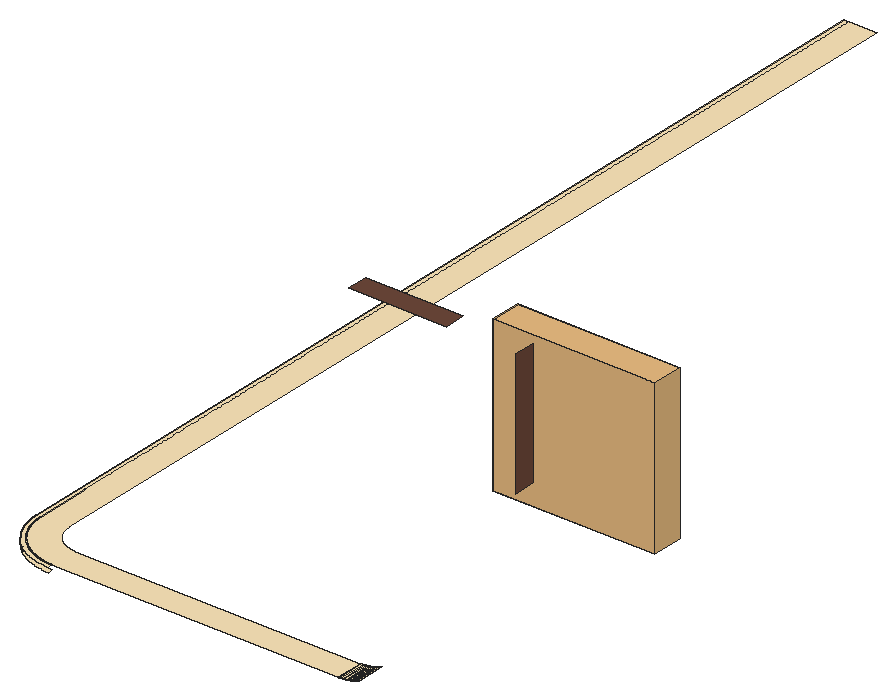
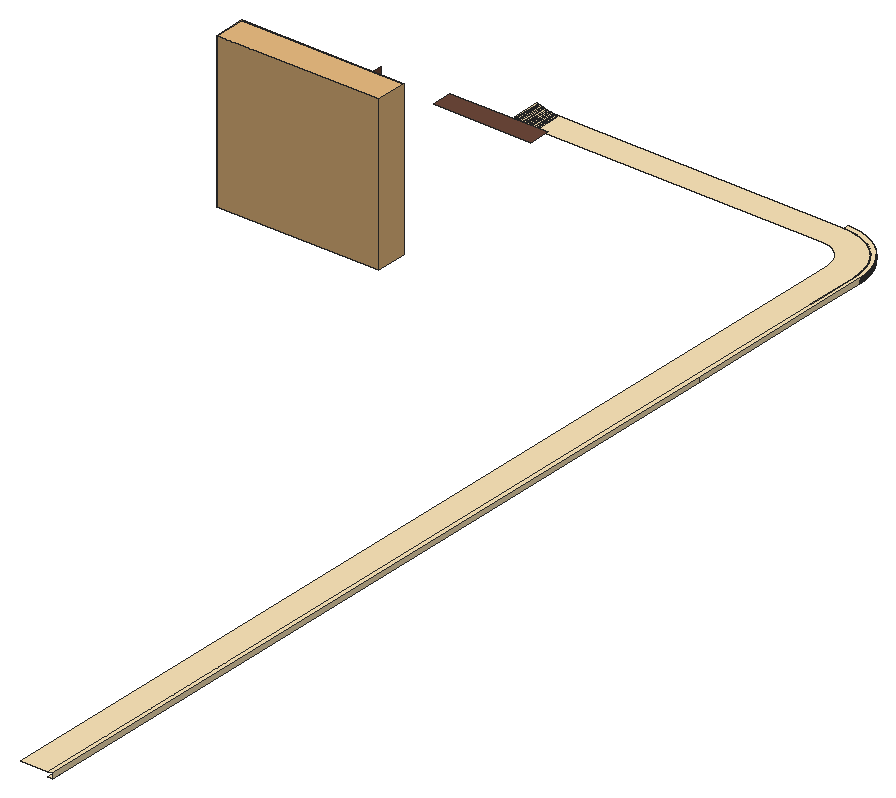
# SketchUp Ruby script. Lengths in inches.
U = 1.inch
M = Sketchup.active_model
def pt(a) = Geom::Point3d.new(a.map { |v| v * U })
def face(e, loops, mat)
  f = e.add_face(loops[0].map { |a| pt(a) })
  loops[1..].each { |l| e.add_face(l.map { |a| pt(a) }).erase! }
  f.material = f.back_material = mat if mat
  f
end
# faces: each face lists its corners as indices into pts; further lists are holes
def faces(e, pts, list, mat = nil) = list.each { |f| face(e, (f[0].is_a?(Array) ? f : [f]).map { |l| l.map { |i| pts[i] } }, mat) }
# xy, xz, yz: faces in a plane at the given z, y or x. An outline is a flat list of corners, or four numbers for a rectangle; further outlines are holes
def ring(l) = l.size == 4 ? [[l[0], l[1]], [l[2], l[1]], [l[2], l[3]], [l[0], l[3]]] : l.each_slice(2).to_a
def flat(e, list, mat, &to3) = list.each { |f| face(e, (f[0].is_a?(Array) ? f : [f]).map { |l| ring(l).map { |u, v| to3.(u, v) } }, mat) }
def xy(e, z, list, mat = nil) = flat(e, list, mat) { |x, y| [x, y, z] }
def xz(e, y, list, mat = nil) = flat(e, list, mat) { |x, z| [x, y, z] }
def yz(e, x, list, mat = nil) = flat(e, list, mat) { |y, z| [x, y, z] }
def lines(e, pts, list) = list.each { |a, b| e.add_line(pt(pts[a]), pt(pts[b])) }
# prism: a flat outline (further loops are holes) pulled along v
def prism(e, loops, v, mat = nil)
  f = face(e, loops, mat); d = Geom::Vector3d.new(v.map { |x| x * U })
  f.pushpull(f.normal.samedirection?(d) ? d.length : -d.length)
end
def box(e, o, s, mat = nil) = prism(e, [[o, [o[0] + s[0], o[1], o[2]], [o[0] + s[0], o[1] + s[1], o[2]], [o[0], o[1] + s[1], o[2]]]], [0, 0, s[2]], mat)
def at(x, y, z, deg = 0) = Geom::Transformation.translation(pt([x, y, z])) * Geom::Transformation.rotation(ORIGIN, Z_AXIS, deg.degrees)
def axes(o, x, y, z) = Geom::Transformation.new([*x, 0, *y, 0, *z, 0, *pt(o).to_a, 1])
def part(name) = M.definitions.add(name)
# library, detail: a bought-in or finely detailed component or shape, given as its bounding box
def library(name, o, s) = part(name).tap { |d| box(d.entities, o, s) }
def detail(e, o, s) = box(e.add_group.entities, o, s)
def put(e, d, t, mat = nil) = e.add_instance(d, t).tap { |i| i.material = mat if mat }
def group(e, t, mat = nil) = e.add_group.tap { |g| g.transformation = t; g.material = mat if mat }.entities
root = M.entities
M.materials.add("1026 AP 7946 SUNNY SIDE UP").color = [254, 231, 186]
M.materials.add("1916 AP K226 Macadamia Cream-N").color = [109, 72, 58]
c1 = library("---------1\#1",[5.49,6.625,-77.21],[69.81,13.39,114.05])
xy(root,142,[[29.49,213.1,28.99,213.12,28.73,213.13,28.48,213.14,27.98,213.18,27.72,213.2,27.47,213.22,26.72,213.31,26.46,213.34,25.46,213.5,25.21,213.55,24.97,213.59,24.72,213.65,24.22,213.75,23.98,213.8125,23.73,213.87,23.48,213.93,23.24,214,22.99,214.07,22.27,214.28,22.02,214.36,21.54,214.52,21.31,214.61,21.07,214.69,20.59,214.87,20.36,214.97,20.125,215.0625,19.89,215.16,19.43,215.36,19.19,215.47,18.96,215.57,18.74,215.68,18.51,215.8,18.28,215.91,18.06,216.02,17.83,216.14,17.61,216.26,17.39,216.39,17.17,216.51,16.51,216.9,16.3,217.03,16.08,217.17,15.87,217.3,15.66,217.44,15.45,217.59,15.24,217.73,15.03,217.875,14.83,218.02,14.42,218.32,14.22,218.48,14.02,218.63,13.82,218.79,13.43,219.11,13.24,219.28,13.04,219.44,12.66,219.78,12.48,219.95,12.29,220.12,12.11,220.3,11.93,220.47,11.39,221.01,11.22,221.2,11.04,221.38,10.53,221.95,10.21,222.33,10.04,222.53,9.88,222.72,9.73,222.92,9.57,223.12,9.42,223.32,9.26,223.52,9.11,223.73,8.96,223.93,8.82,224.14,8.67,224.35,8.25,224.98,8.12,225.2,7.99,225.41,7.85,225.63,7.72,225.84,7.6,226.0625,7.47,226.28,7.35,226.51,7.11,226.95,6.99,227.18,6.88,227.4,6.44,228.32,6.24,228.78,6.14,229.02,6.05,229.25,5.95,229.49,5.86,229.72,5.68,230.2,5.6,230.4375,5.52,230.68,5.4375,230.92,5.36,231.16,5.29,231.4,5.21,231.64,5.14,231.89,5.07,232.13,4.95,232.62,4.88,232.87,4.83,233.11,4.77,233.36,4.67,233.86,4.62,234.1,4.57,234.35,4.41,235.35,4.38,235.61,4.29,236.36,4.27,236.61,4.24,236.87,4.23,237.12,4.21,237.37,4.19,237.625,4.18,237.875,4.17,238.13,4.17,238.38,4.16,238.64,4.12,262.95,6,262.9375,6.16,238.66,6.17,238.43,6.17,238.19,6.19,237.73,6.21,237.49,6.22,237.26,6.24,237.03,6.26,236.79,6.3,236.33,6.33,236.1,6.36,235.86,6.39,235.63,6.43,235.4,6.46,235.17,6.5,234.9375,6.54,234.71,6.58,234.48,6.67,234.02,6.72,233.79,6.77,233.5625,6.83,233.34,6.88,233.11,6.94,232.88,7,232.66,7.07,232.43,7.13,232.21,7.2,231.98,7.41,231.32,7.49,231.09,7.57,230.875,7.65,230.65,7.73,230.4375,7.8125,230.22,7.9,230,7.99,229.78,8.08,229.57,8.17,229.35,8.27,229.14,8.36,228.93,8.56,228.51,8.67,228.3,8.77,228.09,8.99,227.67,9.1,227.47,9.22,227.26,9.33,227.06,9.57,226.66,9.6875,226.46,9.8125,226.26,9.9375,226.0625,10.07,225.87,10.19,225.67,10.33,225.48,10.46,225.28,10.59,225.09,10.73,224.9,10.87,224.72,11.15,224.34,11.29,224.16,11.74,223.62,11.89,223.4375,12.04,223.26,12.2,223.09,12.35,222.91,12.99,222.23,13.16,222.07,13.49,221.74,13.83,221.42,14.01,221.26,14.18,221.1,14.36,220.95,14.53,220.8,15.07,220.35,15.26,220.21,15.44,220.0625,15.625,219.92,16,219.64,16.19,219.51,16.38,219.37,16.58,219.24,16.96,218.98,17.16,218.85,17.36,218.73,17.56,218.6,17.96,218.36,18.16,218.25,18.36,218.13,18.57,218.02,18.77,217.91,18.98,217.8,19.1875,217.69,19.4,217.59,19.61,217.48,20.03,217.28,20.24,217.1875,20.46,217.09,20.67,217,20.89,216.91,21.1,216.82,21.32,216.74,21.54,216.65,22.2,216.41,22.42,216.34,22.64,216.26,22.86,216.19,23.09,216.125,23.3125,216.06,23.54,215.99,23.76,215.93,23.99,215.87,24.21,215.8125,24.44,215.76,24.67,215.7,24.9,215.65,25.125,215.6,25.35,215.56,25.58,215.51,25.8125,215.47,26.04,215.43,26.28,215.39,26.51,215.36,26.74,215.32,27.2,215.26,27.43,215.24,27.67,215.21,28.13,215.17,28.36,215.16,28.6,215.14,28.83,215.13,29.07,215.12,29.53,215.1,29.77,215.1,29.76,215,29.75,213.1],[6,262.9375,4.12,262.95,4,325.89,4,674,6,674]],"1026 AP 7946 SUNNY SIDE UP")
xy(root,144,[[29.49,213.1,29.75,213.1,29.76,215,29.53,215,29.29,215.01,29.06,215.02,28.82,215.03,28.59,215.04,28.35,215.06,28.12,215.07,27.88,215.09,27.65,215.12,27.42,215.14,27.18,215.17,26.95,215.19,26.72,215.23,26.48,215.26,26.25,215.29,25.79,215.37,25.55,215.42,25.32,215.46,24.4,215.66,24.18,215.72,23.49,215.9,23.27,215.96,23.04,216.03,22.82,216.1,22.59,216.17,22.37,216.25,22.15,216.32,21.92,216.4,21.7,216.48,21.48,216.5625,21.26,216.65,21.04,216.73,20.83,216.82,20.61,216.91,20.39,217.01,20.18,217.1,19.96,217.2,19.33,217.5,18.7,217.83,18.49,217.9375,18.29,218.05,18.08,218.17,17.67,218.41,17.27,218.65,17.07,218.78,16.68,219.04,16.48,219.17,16.29,219.3,16.1,219.4375,15.91,219.57,15.53,219.85,15.34,220,15.16,220.14,14.97,220.29,14.25,220.89,14.07,221.05,13.9,221.2,13.72,221.36,13.38,221.68,13.21,221.85,13.04,222.01,12.88,222.18,12.71,222.35,12.39,222.69,12.23,222.87,12.08,223.04,11.92,223.22,11.77,223.39,11.61,223.57,11.46,223.76,11.31,223.9375,11.17,224.12,11.02,224.31,10.88,224.49,10.6,224.87,10.46,225.0625,10.33,225.25,10.19,225.45,10.06,225.64,9.8,226.04,9.68,226.24,9.55,226.44,9.19,227.04,9.07,227.25,8.96,227.45,8.52,228.29,8.22,228.92,8.12,229.14,8.02,229.35,7.93,229.57,7.84,229.78,7.66,230.22,7.58,230.44,7.49,230.66,7.41,230.88,7.34,231.1,7.26,231.33,7.19,231.55,7.11,231.77,7.04,232,6.98,232.22,6.91,232.45,6.85,232.68,6.79,232.9,6.67,233.36,6.42,234.51,6.34,234.97,6.3,235.21,6.27,235.4375,6.23,235.67,6.2,235.9,6.17,236.14,6.14,236.37,6.12,236.61,6.1,236.84,6.08,237.08,6.04,237.54,6.03,237.78,6.02,238.01,6,238.49,6,674,4,674,4,325.89,4.16,238.64,4.17,238.38,4.17,238.13,4.18,237.875,4.19,237.625,4.21,237.37,4.23,237.12,4.24,236.87,4.27,236.61,4.29,236.36,4.38,235.61,4.41,235.35,4.57,234.35,4.62,234.1,4.67,233.86,4.77,233.36,4.83,233.11,4.88,232.87,4.95,232.62,5.07,232.13,5.14,231.89,5.21,231.64,5.29,231.4,5.36,231.16,5.4375,230.92,5.52,230.68,5.6,230.4375,5.68,230.2,5.86,229.72,5.95,229.49,6.05,229.25,6.14,229.02,6.24,228.78,6.44,228.32,6.88,227.4,6.99,227.18,7.11,226.95,7.35,226.51,7.47,226.28,7.6,226.0625,7.72,225.84,7.85,225.63,7.99,225.41,8.12,225.2,8.25,224.98,8.67,224.35,8.82,224.14,8.96,223.93,9.11,223.73,9.26,223.52,9.42,223.32,9.57,223.12,9.73,222.92,9.88,222.72,10.04,222.53,10.21,222.33,10.53,221.95,11.04,221.38,11.22,221.2,11.39,221.01,11.93,220.47,12.11,220.3,12.29,220.12,12.48,219.95,12.66,219.78,13.04,219.44,13.24,219.28,13.43,219.11,13.82,218.79,14.02,218.63,14.22,218.48,14.42,218.32,14.83,218.02,15.03,217.875,15.24,217.73,15.45,217.59,15.66,217.44,15.87,217.3,16.08,217.17,16.3,217.03,16.51,216.9,17.17,216.51,17.39,216.39,17.61,216.26,17.83,216.14,18.06,216.02,18.28,215.91,18.51,215.8,18.74,215.68,18.96,215.57,19.19,215.47,19.43,215.36,19.89,215.16,20.125,215.0625,20.36,214.97,20.59,214.87,21.07,214.69,21.31,214.61,21.54,214.52,22.02,214.36,22.27,214.28,22.99,214.07,23.24,214,23.48,213.93,23.73,213.87,23.98,213.8125,24.22,213.75,24.72,213.65,24.97,213.59,25.21,213.55,25.46,213.5,26.46,213.34,26.72,213.31,27.47,213.22,27.72,213.2,27.98,213.18,28.48,213.14,28.73,213.13,28.99,213.12],[29.53,215,29.76,215,29.77,215.1,29.53,215.1,29.07,215.12,28.83,215.13,28.6,215.14,28.36,215.16,28.13,215.17,27.67,215.21,27.43,215.24,27.2,215.26,26.74,215.32,26.51,215.36,26.28,215.39,26.04,215.43,25.8125,215.47,25.58,215.51,25.35,215.56,25.125,215.6,24.9,215.65,24.67,215.7,24.44,215.76,24.21,215.8125,23.99,215.87,23.76,215.93,23.54,215.99,23.3125,216.06,23.09,216.125,22.86,216.19,22.64,216.26,22.42,216.34,22.2,216.41,21.54,216.65,21.32,216.74,21.1,216.82,20.89,216.91,20.67,217,20.46,217.09,20.24,217.1875,20.03,217.28,19.61,217.48,19.4,217.59,19.1875,217.69,18.98,217.8,18.77,217.91,18.57,218.02,18.36,218.13,18.16,218.25,17.96,218.36,17.56,218.6,17.36,218.73,17.16,218.85,16.96,218.98,16.58,219.24,16.38,219.37,16.19,219.51,16,219.64,15.625,219.92,15.44,220.0625,15.26,220.21,15.07,220.35,14.53,220.8,14.36,220.95,14.18,221.1,14.01,221.26,13.83,221.42,13.49,221.74,13.16,222.07,12.99,222.23,12.35,222.91,12.2,223.09,12.04,223.26,11.89,223.4375,11.74,223.62,11.29,224.16,11.15,224.34,10.87,224.72,10.73,224.9,10.59,225.09,10.46,225.28,10.33,225.48,10.19,225.67,10.07,225.87,9.9375,226.0625,9.8125,226.26,9.6875,226.46,9.57,226.66,9.33,227.06,9.22,227.26,9.1,227.47,8.99,227.67,8.77,228.09,8.67,228.3,8.56,228.51,8.36,228.93,8.27,229.14,8.17,229.35,8.08,229.57,7.99,229.78,7.9,230,7.8125,230.22,7.73,230.4375,7.65,230.65,7.57,230.875,7.49,231.09,7.41,231.32,7.2,231.98,7.13,232.21,7.07,232.43,7,232.66,6.94,232.88,6.88,233.11,6.83,233.34,6.77,233.5625,6.72,233.79,6.67,234.02,6.58,234.48,6.54,234.71,6.5,234.9375,6.46,235.17,6.43,235.4,6.39,235.63,6.36,235.86,6.33,236.1,6.3,236.33,6.26,236.79,6.24,237.03,6.22,237.26,6.21,237.49,6.19,237.73,6.17,238.19,6.17,238.43,6.16,238.66,6,262.9375,6,238.49,6.02,238.01,6.03,237.78,6.04,237.54,6.08,237.08,6.1,236.84,6.12,236.61,6.14,236.37,6.17,236.14,6.2,235.9,6.23,235.67,6.27,235.4375,6.3,235.21,6.34,234.97,6.42,234.51,6.67,233.36,6.79,232.9,6.85,232.68,6.91,232.45,6.98,232.22,7.04,232,7.11,231.77,7.19,231.55,7.26,231.33,7.34,231.1,7.41,230.88,7.49,230.66,7.58,230.44,7.66,230.22,7.84,229.78,7.93,229.57,8.02,229.35,8.12,229.14,8.22,228.92,8.52,228.29,8.96,227.45,9.07,227.25,9.19,227.04,9.55,226.44,9.68,226.24,9.8,226.04,10.06,225.64,10.19,225.45,10.33,225.25,10.46,225.0625,10.6,224.87,10.88,224.49,11.02,224.31,11.17,224.12,11.31,223.9375,11.46,223.76,11.61,223.57,11.77,223.39,11.92,223.22,12.08,223.04,12.23,222.87,12.39,222.69,12.71,222.35,12.88,222.18,13.04,222.01,13.21,221.85,13.38,221.68,13.72,221.36,13.9,221.2,14.07,221.05,14.25,220.89,14.97,220.29,15.16,220.14,15.34,220,15.53,219.85,15.91,219.57,16.1,219.4375,16.29,219.3,16.48,219.17,16.68,219.04,17.07,218.78,17.27,218.65,17.67,218.41,18.08,218.17,18.29,218.05,18.49,217.9375,18.7,217.83,19.33,217.5,19.96,217.2,20.18,217.1,20.39,217.01,20.61,216.91,20.83,216.82,21.04,216.73,21.26,216.65,21.48,216.5625,21.7,216.48,21.92,216.4,22.15,216.32,22.37,216.25,22.59,216.17,22.82,216.1,23.04,216.03,23.27,215.96,23.49,215.9,24.18,215.72,24.4,215.66,25.32,215.46,25.55,215.42,25.79,215.37,26.25,215.29,26.48,215.26,26.72,215.23,26.95,215.19,27.18,215.17,27.42,215.14,27.65,215.12,27.88,215.09,28.12,215.07,28.35,215.06,28.59,215.04,28.82,215.03,29.06,215.02,29.29,215.01],[29.53,215.1,153,215.1,153,227,29.81,227,29.53,227.01,29.29,227.02,29.06,227.04,28.82,227.06,28.59,227.08,28.36,227.11,28.01,227.17,27.77,227.21,27.54,227.25,27.3125,227.3,27.08,227.36,26.86,227.42,26.63,227.48,26.52,227.52,26.18,227.625,25.96,227.7,25.74,227.78,25.08,228.05,24.66,228.25,24.24,228.47,24.03,228.59,23.63,228.83,23.43,228.96,23.24,229.09,23.04,229.22,22.66,229.5,22.48,229.65,22.39,229.72,22.03,230.03,21.85,230.1875,21.68,230.35,21.35,230.68,21.1875,230.85,21.03,231.03,20.72,231.39,20.58,231.57,20.43,231.76,20.36,231.85,20.22,232.04,20.15,232.14,20.02,232.33,19.89,232.53,19.65,232.93,19.53,233.14,19.47,233.24,19.36,233.45,19.2,233.76,19.15,233.87,19.05,234.08,18.78,234.74,18.66,235.07,18.55,235.4,18.52,235.52,18.45,235.74,18.42,235.86,18.36,236.08,18.3,236.3125,18.25,236.54,18.23,236.66,18.1875,236.89,18.17,237.01,18.11,237.36,18.08,237.59,18.06,237.82,18.04,238.06,18.02,238.29,18.01,238.53,18,238.76,18,674,6,674,6,262.9375,6.16,238.66,6.17,238.43,6.17,238.19,6.19,237.73,6.21,237.49,6.22,237.26,6.24,237.03,6.26,236.79,6.3,236.33,6.33,236.1,6.36,235.86,6.39,235.63,6.43,235.4,6.46,235.17,6.5,234.9375,6.54,234.71,6.58,234.48,6.67,234.02,6.72,233.79,6.77,233.5625,6.83,233.34,6.88,233.11,6.94,232.88,7,232.66,7.07,232.43,7.13,232.21,7.2,231.98,7.41,231.32,7.49,231.09,7.57,230.875,7.65,230.65,7.73,230.4375,7.8125,230.22,7.9,230,7.99,229.78,8.08,229.57,8.17,229.35,8.27,229.14,8.36,228.93,8.56,228.51,8.67,228.3,8.77,228.09,8.99,227.67,9.1,227.47,9.22,227.26,9.33,227.06,9.57,226.66,9.6875,226.46,9.8125,226.26,9.9375,226.0625,10.07,225.87,10.19,225.67,10.33,225.48,10.46,225.28,10.59,225.09,10.73,224.9,10.87,224.72,11.15,224.34,11.29,224.16,11.74,223.62,11.89,223.4375,12.04,223.26,12.2,223.09,12.35,222.91,12.99,222.23,13.16,222.07,13.49,221.74,13.83,221.42,14.01,221.26,14.18,221.1,14.36,220.95,14.53,220.8,15.07,220.35,15.26,220.21,15.44,220.0625,15.625,219.92,16,219.64,16.19,219.51,16.38,219.37,16.58,219.24,16.96,218.98,17.16,218.85,17.36,218.73,17.56,218.6,17.96,218.36,18.16,218.25,18.36,218.13,18.57,218.02,18.77,217.91,18.98,217.8,19.1875,217.69,19.4,217.59,19.61,217.48,20.03,217.28,20.24,217.1875,20.46,217.09,20.67,217,20.89,216.91,21.1,216.82,21.32,216.74,21.54,216.65,22.2,216.41,22.42,216.34,22.64,216.26,22.86,216.19,23.09,216.125,23.3125,216.06,23.54,215.99,23.76,215.93,23.99,215.87,24.21,215.8125,24.44,215.76,24.67,215.7,24.9,215.65,25.125,215.6,25.35,215.56,25.58,215.51,25.8125,215.47,26.04,215.43,26.28,215.39,26.51,215.36,26.74,215.32,27.2,215.26,27.43,215.24,27.67,215.21,28.13,215.17,28.36,215.16,28.6,215.14,28.83,215.13,29.07,215.12],[153,215.1,153.24,227],[153.24,215.1,153.47,227]],"1026 AP 7946 SUNNY SIDE UP")
xy(root,216,[[69,326,111,335]],"1916 AP K226 Macadamia Cream-N")
yz(root,4,[[325.89,142,674,144]],"1026 AP 7946 SUNNY SIDE UP")
yz(root,4.17,[[238.13,142,238.38,144]],"1026 AP 7946 SUNNY SIDE UP")
yz(root,6.17,[[238.19,142,238.43,144]],"1026 AP 7946 SUNNY SIDE UP")
yz(root,141,[[326,162,335,216]],"1916 AP K226 Macadamia Cream-N")
p = [[17.96,218.36,142],[17.96,218.36,144],[18.16,218.25,144],[18.16,218.25,142],[14.22,218.48,144],[14.22,218.48,142],
  [14.42,218.32,142],[14.42,218.32,144],[17.76,218.48,142],[17.76,218.48,144],[14.02,218.63,144],[14.02,218.63,142],
  [17.56,218.6,142],[17.56,218.6,144],[13.82,218.79,144],[13.82,218.79,142],[17.36,218.73,142],[17.36,218.73,144],
  [17.16,218.85,142],[17.16,218.85,144],[13.625,218.95,144],[13.625,218.95,142],[16.96,218.98,142],[16.96,218.98,144],
  [13.43,219.11,144],[13.43,219.11,142],[16.77,219.11,142],[16.77,219.11,144],[13.24,219.28,144],[13.24,219.28,142],
  [16.58,219.24,142],[16.58,219.24,144],[16.38,219.37,142],[16.38,219.37,144],[13.04,219.44,144],[13.04,219.44,142],
  [12.85,219.61,144],[12.85,219.61,142],[16.19,219.51,142],[16.19,219.51,144],[16,219.64,142],[16,219.64,144],
  [12.66,219.78,144],[12.66,219.78,142],[15.8125,219.78,142],[15.8125,219.78,144],[12.48,219.95,144],[12.48,219.95,142],
  [15.625,219.92,142],[15.625,219.92,144],[12.29,220.12,144],[12.29,220.12,142],[15.44,220.0625,142],[15.44,220.0625,144],
  [12.11,220.3,144],[12.11,220.3,142],[15.26,220.21,142],[15.26,220.21,144],[15.07,220.35,142],[15.07,220.35,144],
  [11.93,220.47,144],[11.93,220.47,142],[14.89,220.5,142],[14.89,220.5,144],[11.75,220.65,144],[11.75,220.65,142],
  [14.71,220.65,142],[14.71,220.65,144],[14.53,220.8,142],[14.53,220.8,144],[11.57,220.83,144],[11.57,220.83,142],
  [11.39,221.01,144],[11.39,221.01,142],[14.36,220.95,142],[14.36,220.95,144],[11.22,221.2,144],[11.22,221.2,142],
  [14.18,221.1,142],[14.18,221.1,144],[14.01,221.26,142],[14.01,221.26,144],[11.04,221.38,144],[11.04,221.38,142],
  [13.83,221.42,142],[13.83,221.42,144],[10.87,221.57,144],[10.87,221.57,142],[13.66,221.58,142],[13.66,221.58,144],
  [10.7,221.76,144],[10.7,221.76,142],[13.49,221.74,142],[13.49,221.74,144],[13.33,221.9,142],[13.33,221.9,144],
  [10.53,221.95,144],[10.53,221.95,142],[10.37,222.14,144],[10.37,222.14,142],[13.16,222.07,142],[13.16,222.07,144],
  [10.21,222.33,144],[10.21,222.33,142],[12.99,222.23,142],[12.99,222.23,144],[12.83,222.4,142],[12.83,222.4,144],
  [10.04,222.53,144],[10.04,222.53,142],[12.67,222.57,142],[12.67,222.57,144],[9.88,222.72,144],[9.88,222.72,142],
  [12.51,222.74,142],[12.51,222.74,144],[9.73,222.92,144],[9.73,222.92,142],[12.35,222.91,142],[12.35,222.91,144],
  [9.57,223.12,144],[9.57,223.12,142],[12.2,223.09,142],[12.2,223.09,144],[9.42,223.32,144],[9.42,223.32,142],
  [12.04,223.26,142],[12.04,223.26,144],[9.26,223.52,144],[9.26,223.52,142],[11.89,223.4375,142],[11.89,223.4375,144],
  [11.74,223.62,142],[11.74,223.62,144],[9.11,223.73,144],[9.11,223.73,142],[11.59,223.8,142],[11.59,223.8,144],
  [8.96,223.93,144],[8.96,223.93,142],[11.44,223.98,142],[11.44,223.98,144],[8.82,224.14,144],[8.82,224.14,142],
  [11.29,224.16,142],[11.29,224.16,144],[8.67,224.35,144],[8.67,224.35,142],[11.15,224.34,142],[11.15,224.34,144],
  [8.53,224.56,144],[8.53,224.56,142],[11.01,224.53,142],[11.01,224.53,144],[10.87,224.72,142],[10.87,224.72,144],
  [8.39,224.77,144],[8.39,224.77,142],[10.73,224.9,142],[10.73,224.9,144],[8.25,224.98,144],[8.25,224.98,142],
  [10.59,225.09,142],[10.59,225.09,144],[8.12,225.2,144],[8.12,225.2,142],[10.46,225.28,142],[10.46,225.28,144],
  [7.99,225.41,144],[7.99,225.41,142],[10.33,225.48,142],[10.33,225.48,144],[7.85,225.63,144],[7.85,225.63,142],
  [10.19,225.67,142],[10.19,225.67,144],[7.72,225.84,144],[7.72,225.84,142],[10.07,225.87,142],[10.07,225.87,144],
  [7.6,226.0625,144],[7.6,226.0625,142],[9.9375,226.0625,142],[9.9375,226.0625,144],[7.47,226.28,144],[7.47,226.28,142],
  [9.8125,226.26,142],[9.8125,226.26,144],[7.35,226.51,144],[7.35,226.51,142],[9.6875,226.46,142],[9.6875,226.46,144],
  [7.23,226.73,144],[7.23,226.73,142],[9.57,226.66,142],[9.57,226.66,144],[7.11,226.95,144],[7.11,226.95,142],
  [9.45,226.86,142],[9.45,226.86,144],[9.33,227.06,142],[9.33,227.06,144],[6.99,227.18,144],[6.99,227.18,142],
  [9.22,227.26,142],[9.22,227.26,144],[6.88,227.4,144],[6.88,227.4,142],[9.1,227.47,142],[9.1,227.47,144],
  [6.77,227.63,144],[6.77,227.63,142],[8.99,227.67,142],[8.99,227.67,144],[6.66,227.86,144],[6.66,227.86,142],
  [8.88,227.88,142],[8.88,227.88,144],[6.55,228.09,144],[6.55,228.09,142],[8.77,228.09,142],[8.77,228.09,144],
  [6.44,228.32,144],[6.44,228.32,142],[8.67,228.3,142],[8.67,228.3,144],[6.34,228.55,144],[6.34,228.55,142],
  [8.56,228.51,142],[8.56,228.51,144],[8.46,228.72,142],[8.46,228.72,144],[6.24,228.78,144],[6.24,228.78,142],
  [8.36,228.93,142],[8.36,228.93,144],[6.14,229.02,144],[6.14,229.02,142],[8.27,229.14,142],[8.27,229.14,144],
  [6.05,229.25,144],[6.05,229.25,142],[8.17,229.35,142],[8.17,229.35,144],[5.95,229.49,144],[5.95,229.49,142],
  [8.08,229.57,142],[8.08,229.57,144],[5.86,229.72,144],[5.86,229.72,142],[7.99,229.78,142],[7.99,229.78,144],
  [5.77,229.96,144],[5.77,229.96,142],[7.9,230,142],[7.9,230,144],[5.68,230.2,144],[5.68,230.2,142],
  [7.8125,230.22,142],[7.8125,230.22,144],[5.6,230.4375,144],[5.6,230.4375,142],[7.73,230.4375,142],[7.73,230.4375,144],
  [5.52,230.68,144],[5.52,230.68,142],[7.65,230.65,142],[7.65,230.65,144],[5.4375,230.92,144],[5.4375,230.92,142],
  [7.57,230.875,142],[7.57,230.875,144],[5.36,231.16,144],[5.36,231.16,142],[7.49,231.09,142],[7.49,231.09,144],
  [7.41,231.32,142],[7.41,231.32,144],[5.29,231.4,144],[5.29,231.4,142],[7.34,231.54,142],[7.34,231.54,144],
  [5.21,231.64,144],[5.21,231.64,142],[7.27,231.76,142],[7.27,231.76,144],[5.14,231.89,144],[5.14,231.89,142],
  [7.2,231.98,142],[7.2,231.98,144],[5.07,232.13,144],[5.07,232.13,142],[7.13,232.21,142],[7.13,232.21,144],
  [5.01,232.375,144],[5.01,232.375,142],[7.07,232.43,142],[7.07,232.43,144],[4.95,232.62,144],[4.95,232.62,142],
  [7,232.66,142],[7,232.66,144],[4.88,232.87,144],[4.88,232.87,142],[6.94,232.88,142],[6.94,232.88,144],
  [4.83,233.11,144],[4.83,233.11,142],[6.88,233.11,142],[6.88,233.11,144],[4.77,233.36,144],[4.77,233.36,142],
  [6.83,233.34,142],[6.83,233.34,144],[6.77,233.5625,142],[6.77,233.5625,144],[4.72,233.61,144],[4.72,233.61,142],
  [4.67,233.86,144],[4.67,233.86,142],[6.72,233.79,142],[6.72,233.79,144],[6.67,234.02,142],[6.67,234.02,144],
  [4.62,234.1,144],[4.62,234.1,142],[6.625,234.25,142],[6.625,234.25,144],[4.57,234.35,144],[4.57,234.35,142],
  [6.58,234.48,142],[6.58,234.48,144],[4.53,234.6,144],[4.53,234.6,142],[6.54,234.71,142],[6.54,234.71,144],
  [4.49,234.85,144],[4.49,234.85,142],[6.5,234.9375,142],[6.5,234.9375,144],[4.45,235.1,144],[4.45,235.1,142],
  [6.46,235.17,142],[6.46,235.17,144],[4.41,235.35,144],[4.41,235.35,142],[6.43,235.4,142],[6.43,235.4,144],
  [4.38,235.61,144],[4.38,235.61,142],[6.39,235.63,142],[6.39,235.63,144],[4.35,235.86,144],[4.35,235.86,142],
  [6.36,235.86,142],[6.36,235.86,144],[4.32,236.11,144],[4.32,236.11,142],[6.33,236.1,142],[6.33,236.1,144],
  [4.29,236.36,144],[4.29,236.36,142],[6.3,236.33,142],[6.3,236.33,144],[6.28,236.56,142],[6.28,236.56,144],
  [4.27,236.61,144],[4.27,236.61,142],[4.24,236.87,144],[4.24,236.87,142],[6.26,236.79,142],[6.26,236.79,144],
  [6.24,237.03,142],[6.24,237.03,144],[4.23,237.12,144],[4.23,237.12,142],[6.22,237.26,142],[6.22,237.26,144],
  [4.21,237.37,144],[4.21,237.37,142],[6.21,237.49,142],[6.21,237.49,144],[4.19,237.625,144],[4.19,237.625,142],
  [6.19,237.73,142],[6.19,237.73,144],[4.18,237.875,144],[4.18,237.875,142],[6.18,237.96,142],[6.18,237.96,144],
  [4.17,238.13,144],[4.17,238.13,142],[6.17,238.19,142],[6.17,238.19,144],[4.16,238.64,144],[4.16,238.64,142],
  [4.17,238.38,142],[4.17,238.38,144],[6.16,238.66,142],[6.16,238.66,144],[6.17,238.43,144],[6.17,238.43,142],
  [4,325.89,144],[4,325.89,142],[4.12,262.95,142],[6,262.9375,142],[6,262.9375,144],[153.47,227,144],
  [153.47,215.1,144],[153.71,215.1,144.01],[153.71,227,144.01],[153.94,215.1,144.02],[153.94,227,144.02],[154.18,215.1,144.03],
  [154.18,227,144.03],[154.41,215.1,144.04],[154.41,227,144.04],[154.65,215.1,144.06],[154.65,227,144.06],[154.88,215.1,144.07],
  [154.88,227,144.07],[155.12,215.1,144.09],[155.12,227,144.09],[155.35,215.1,144.12],[155.35,227,144.12],[155.59,215.1,144.14],
  [155.59,227,144.14],[155.82,215.1,144.17],[155.82,227,144.17],[156.05,215.1,144.2],[156.05,227,144.2],[156.29,215.1,144.23],
  [156.29,227,144.23],[156.52,215.1,144.26],[156.52,227,144.26],[156.75,215.1,144.3],[156.75,227,144.3],[156.99,215.1,144.33],
  [156.99,227,144.33],[157.22,215.1,144.375],[157.22,227,144.375],[157.45,215.1,144.42],[157.45,227,144.42],[157.68,215.1,144.46],
  [157.68,227,144.46],[157.91,215.1,144.51],[157.91,227,144.51],[158.14,215.1,144.56],[158.14,227,144.56],[158.375,215.1,144.61],
  [158.375,227,144.61],[158.6,215.1,144.66],[158.6,227,144.66],[158.83,215.1,144.72],[158.83,227,144.72],[159.06,215.1,144.78],
  [159.06,227,144.78],[159.29,215.1,144.84],[159.29,227,144.84],[159.51,215.1,144.9],[159.51,227,144.9],[159.74,215.1,144.97],
  [159.74,227,144.97],[159.97,215.1,145.03],[159.97,227,145.03],[160.19,215.1,145.1],[160.19,227,145.1],[160.42,215.1,145.17],
  [160.42,227,145.17],[160.64,215.1,145.25],[160.64,227,145.25],[160.86,215.1,145.32],[160.86,227,145.32],[161.09,215.1,145.4],
  [161.09,227,145.4],[161.31,215.1,145.48],[161.31,227,145.48],[161.53,215.1,145.57],[161.53,227,145.57],[161.75,215.1,145.65],
  [161.75,227,145.65],[161.97,215.1,145.74],[161.97,227,145.74],[162.18,215.1,145.83],[162.18,227,145.83]]
faces(root,p,[[0,1,2,3],[4,5,6,7],[8,9,1,0],[10,11,5,4],[12,13,9,8],[14,15,11,10],[16,17,13,12],[18,19,17,16],
  [20,21,15,14],[22,23,19,18],[24,25,21,20],[26,27,23,22],[28,29,25,24],[30,31,27,26],[32,33,31,30],[34,35,29,28],
  [36,37,35,34],[38,39,33,32],[40,41,39,38],[42,43,37,36],[44,45,41,40],[46,47,43,42],[48,49,45,44],[50,51,47,46],
  [52,53,49,48],[54,55,51,50],[56,57,53,52],[58,59,57,56],[60,61,55,54],[62,63,59,58],[64,65,61,60],[66,67,63,62],
  [68,69,67,66],[70,71,65,64],[72,73,71,70],[74,75,69,68],[76,77,73,72],[78,79,75,74],[80,81,79,78],[82,83,77,76],
  [84,85,81,80],[86,87,83,82],[88,89,85,84],[90,91,87,86],[92,93,89,88],[94,95,93,92],[96,97,91,90],[98,99,97,96],
  [100,101,95,94],[102,103,99,98],[104,105,101,100],[106,107,105,104],[108,109,103,102],[110,111,107,106],[112,113,109,108],[114,115,111,110],
  [116,117,113,112],[118,119,115,114],[120,121,117,116],[122,123,119,118],[124,125,121,120],[126,127,123,122],[128,129,125,124],[130,131,127,126],
  [132,133,131,130],[134,135,129,128],[136,137,133,132],[138,139,135,134],[140,141,137,136],[142,143,139,138],[144,145,141,140],[146,147,143,142],
  [148,149,145,144],[150,151,147,146],[152,153,149,148],[154,155,153,152],[156,157,151,150],[158,159,155,154],[160,161,157,156],[162,163,159,158],
  [164,165,161,160],[166,167,163,162],[168,169,165,164],[170,171,167,166],[172,173,169,168],[174,175,171,170],[176,177,173,172],[178,179,175,174],
  [180,181,177,176],[182,183,179,178],[184,185,181,180],[186,187,183,182],[188,189,185,184],[190,191,187,186],[192,193,189,188],[194,195,191,190],
  [196,197,193,192],[198,199,195,194],[200,201,199,198],[202,203,197,196],[204,205,201,200],[206,207,203,202],[208,209,205,204],[210,211,207,206],
  [212,213,209,208],[214,215,211,210],[216,217,213,212],[218,219,215,214],[220,221,217,216],[222,223,219,218],[224,225,221,220],[226,227,223,222],
  [228,229,225,224],[230,231,229,228],[232,233,227,226],[234,235,231,230],[236,237,233,232],[238,239,235,234],[240,241,237,236],[242,243,239,238],
  [244,245,241,240],[246,247,243,242],[248,249,245,244],[250,251,247,246],[252,253,249,248],[254,255,251,250],[256,257,253,252],[258,259,255,254],
  [260,261,257,256],[262,263,259,258],[264,265,261,260],[266,267,263,262],[268,269,265,264],[270,271,267,266],[272,273,269,268],[274,275,271,270],
  [276,277,275,274],[278,279,273,272],[280,281,277,276],[282,283,279,278],[284,285,281,280],[286,287,283,282],[288,289,285,284],[290,291,287,286],
  [292,293,289,288],[294,295,291,290],[296,297,293,292],[298,299,295,294],[300,301,297,296],[302,303,299,298],[304,305,301,300],[306,307,303,302],
  [308,309,305,304],[310,311,307,306],[312,313,309,308],[314,315,313,312],[316,317,311,310],[318,319,317,316],[320,321,315,314],[322,323,321,320],
  [324,325,319,318],[326,327,323,322],[328,329,325,324],[330,331,327,326],[332,333,329,328],[334,335,331,330],[336,337,333,332],[338,339,335,334],
  [340,341,337,336],[342,343,339,338],[344,345,341,340],[346,347,343,342],[348,349,345,344],[350,351,347,346],[352,353,349,348],[354,355,351,350],
  [356,357,353,352],[358,359,355,354],[360,361,357,356],[362,363,359,358],[364,365,363,362],[366,367,361,360],[368,369,367,366],[370,371,365,364],
  [372,373,371,370],[374,375,369,368],[376,377,373,372],[378,379,375,374],[380,381,377,376],[382,383,379,378],[384,385,381,380],[386,387,383,382],
  [388,389,385,384],[390,391,387,386],[392,393,389,388],[394,395,396,397],[398,399,400,401],[402,403,404,395,394],[398,405,406,399],[407,408,409,410],
  [410,409,411,412],[412,411,413,414],[414,413,415,416],[416,415,417,418],[418,417,419,420],[420,419,421,422],[422,421,423,424],[424,423,425,426],
  [426,425,427,428],[428,427,429,430],[430,429,431,432],[432,431,433,434],[434,433,435,436],[436,435,437,438],[438,437,439,440],[440,439,441,442],
  [442,441,443,444],[444,443,445,446],[446,445,447,448],[448,447,449,450],[450,449,451,452],[452,451,453,454],[454,453,455,456],[456,455,457,458],
  [458,457,459,460],[460,459,461,462],[462,461,463,464],[464,463,465,466],[466,465,467,468],[468,467,469,470],[470,469,471,472],[472,471,473,474],
  [474,473,475,476],[476,475,477,478],[478,477,479,480],[480,479,481,482],[482,481,483,484]],"1026 AP 7946 SUNNY SIDE UP")
put(root,c1,axes([118.49,328.375,174.56],[1,0,0],[0,1,0],[0,0,-0.58]),"1026 AP 7946 SUNNY SIDE UP")
